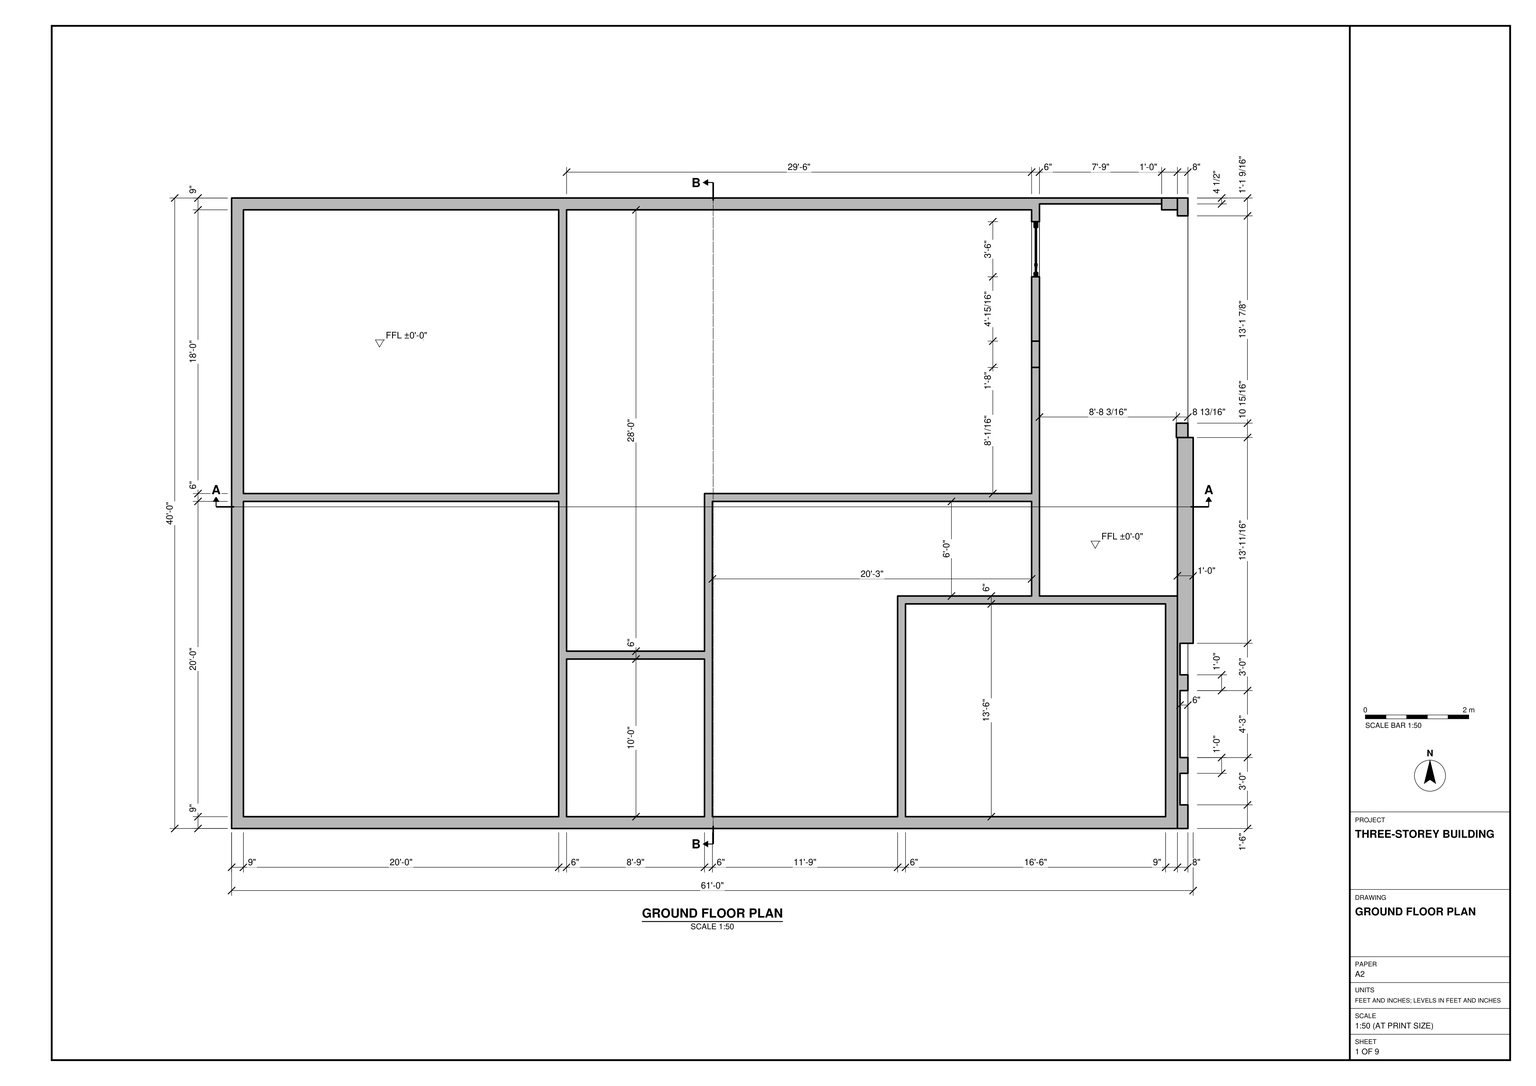
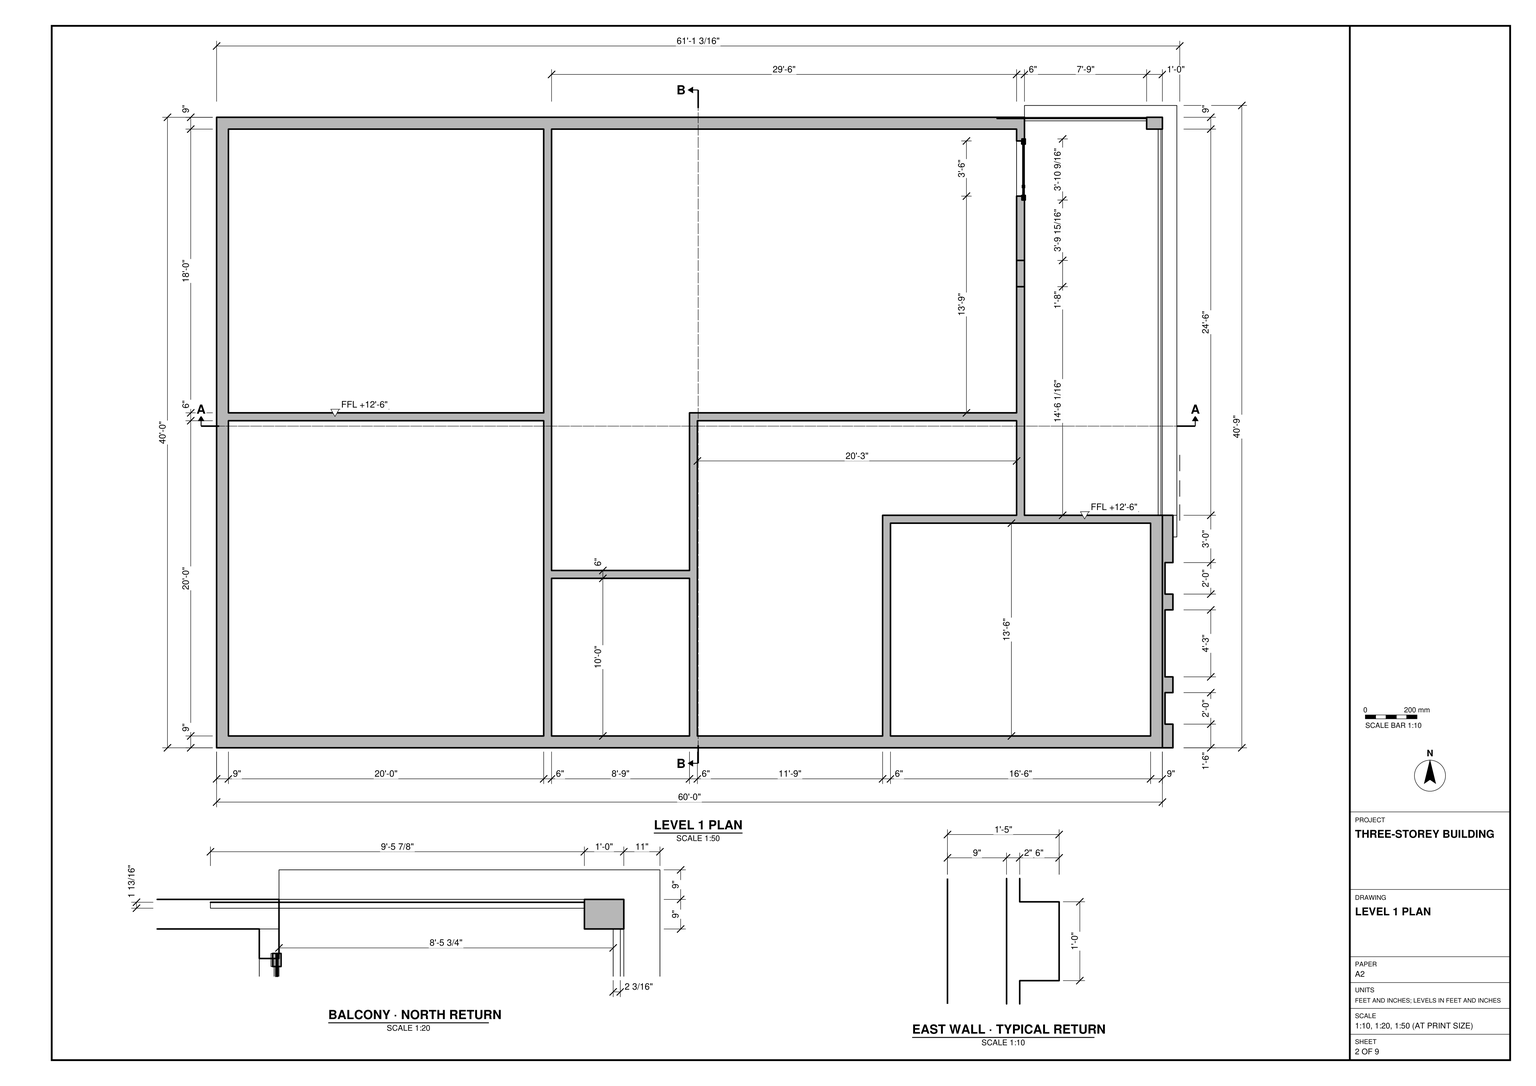
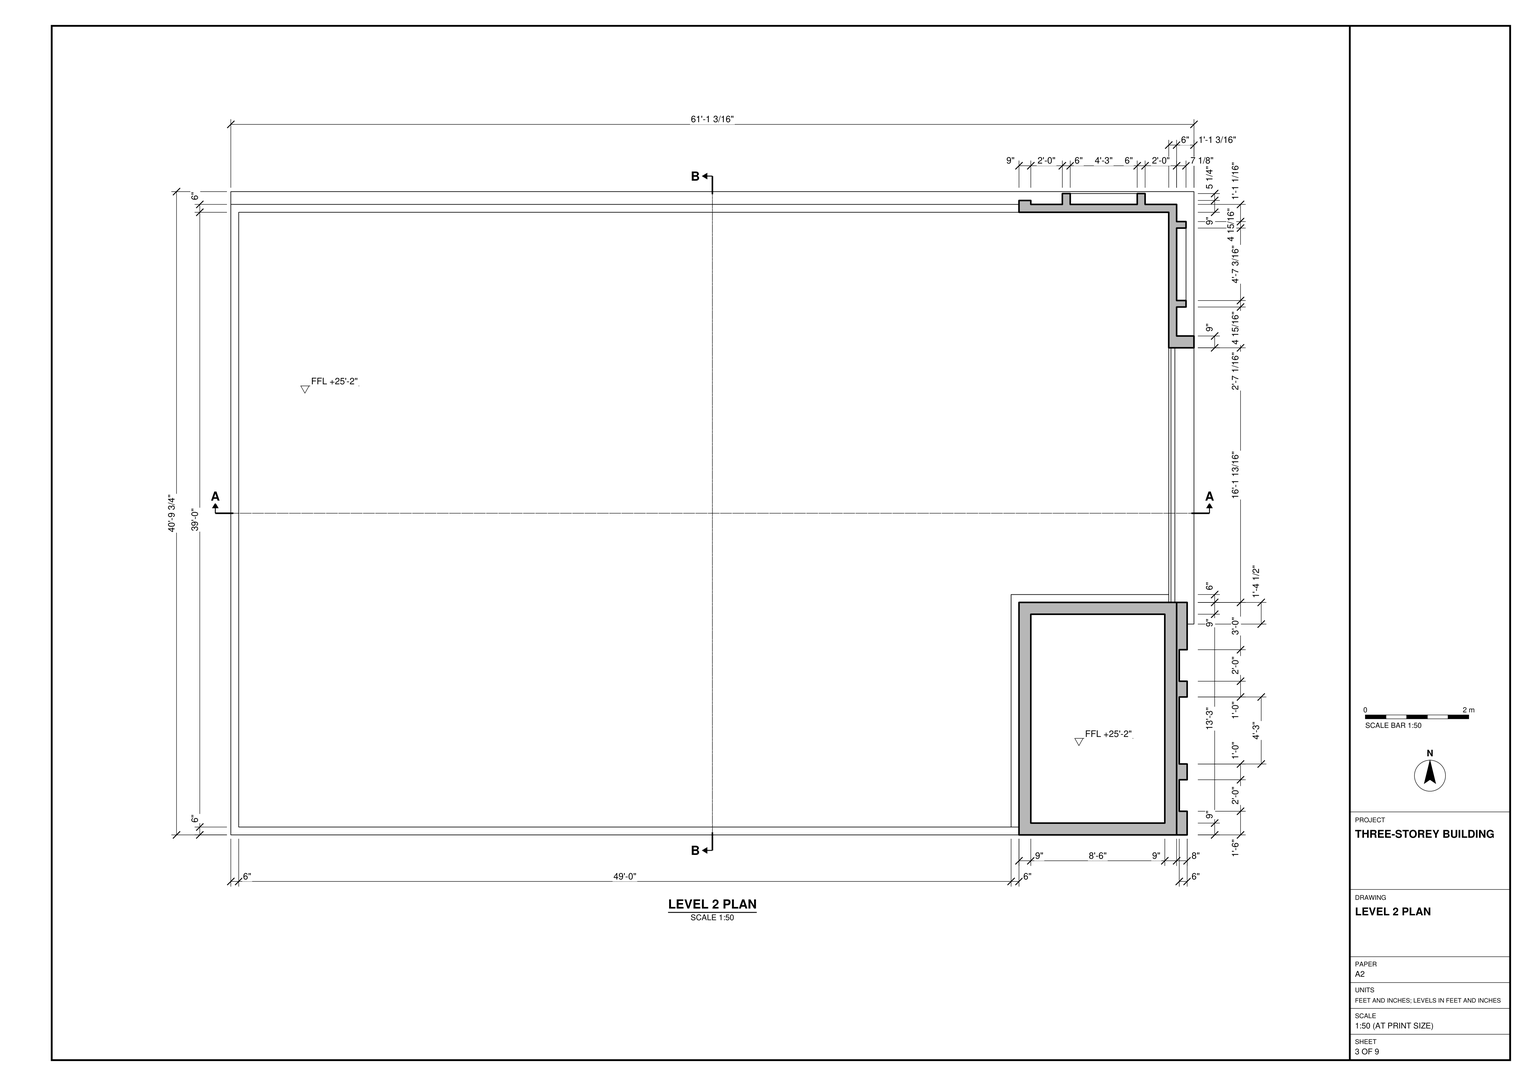
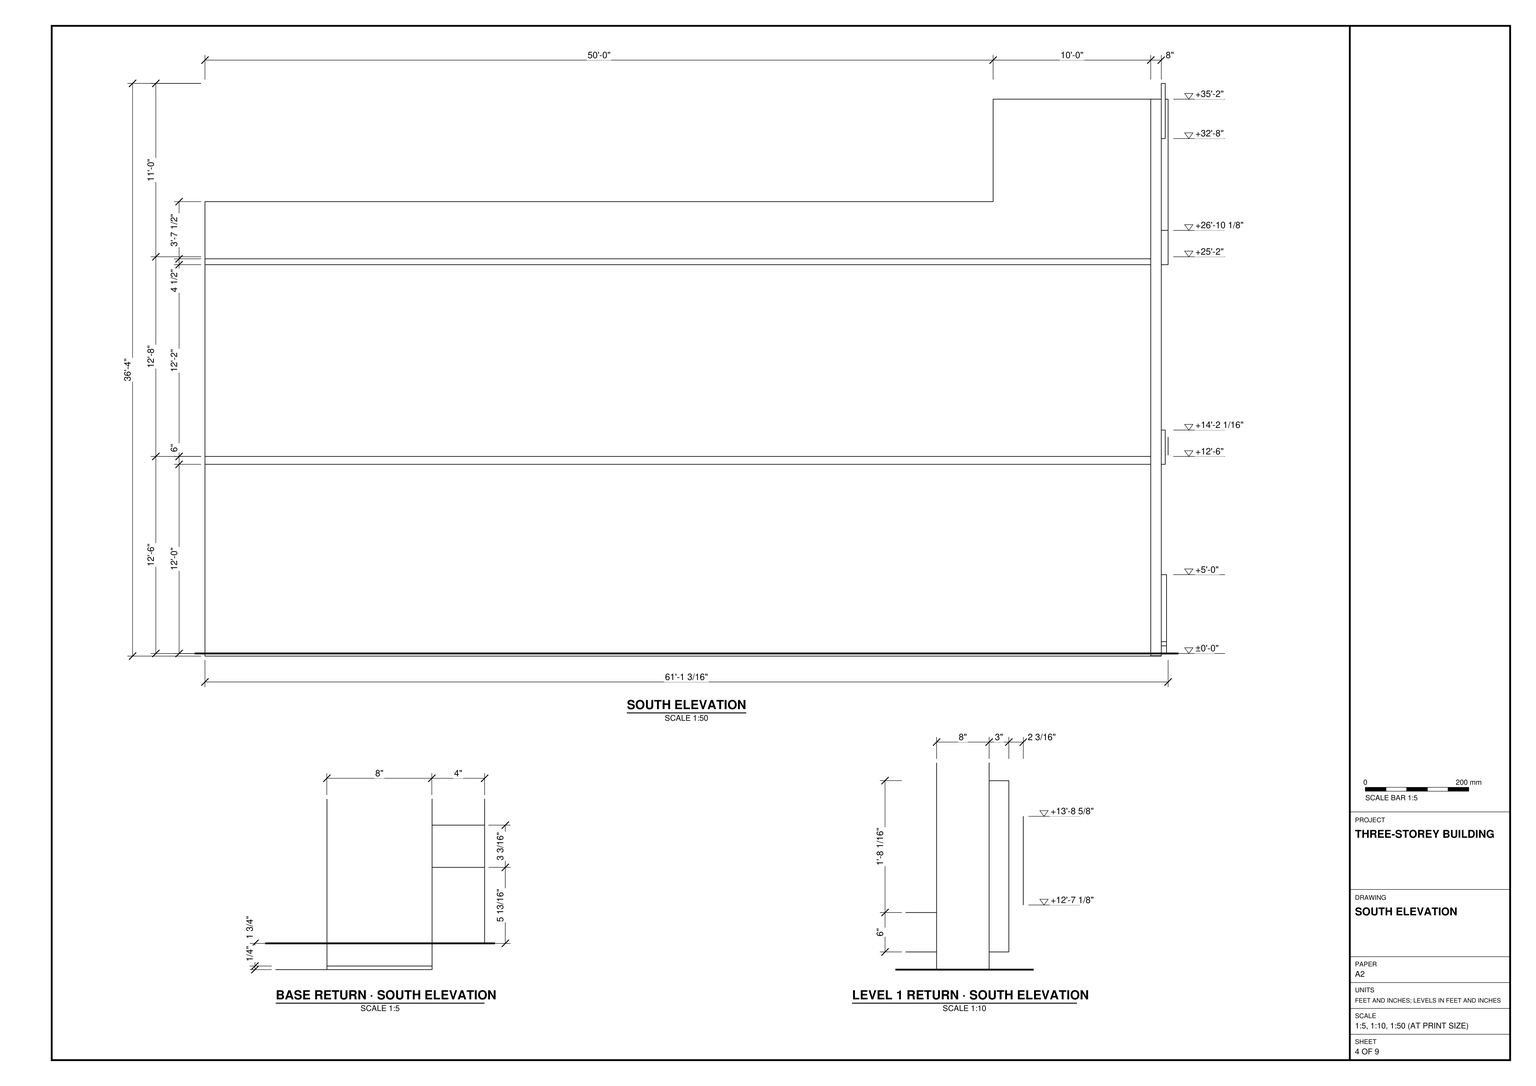
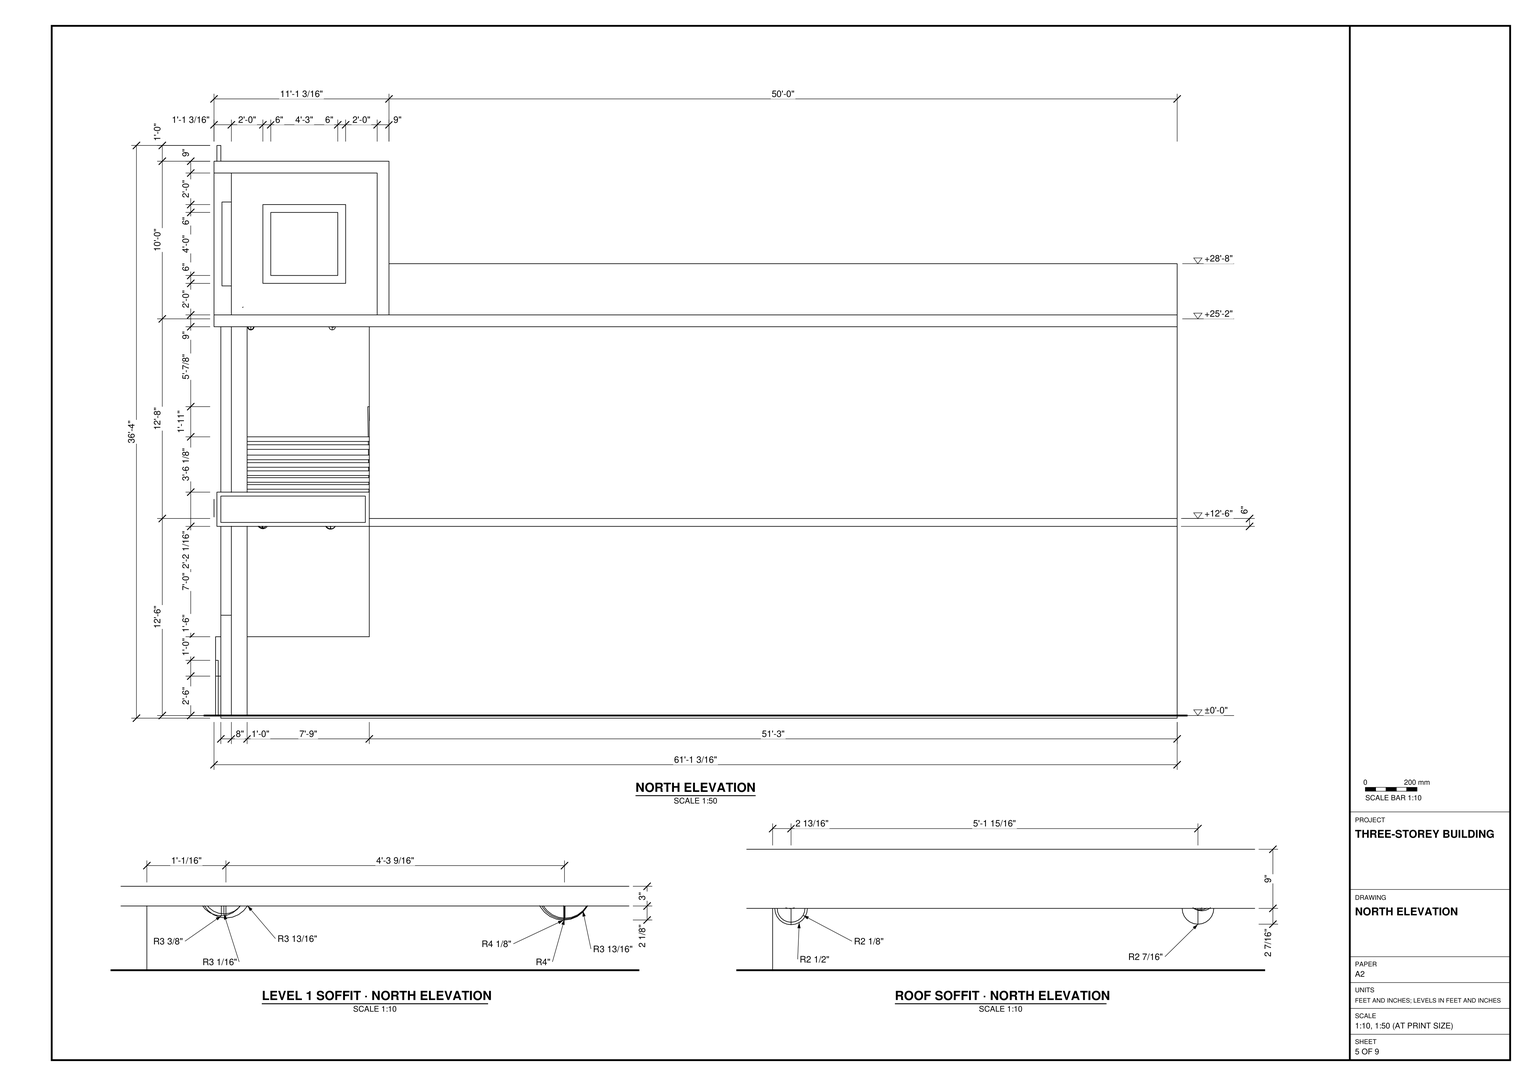
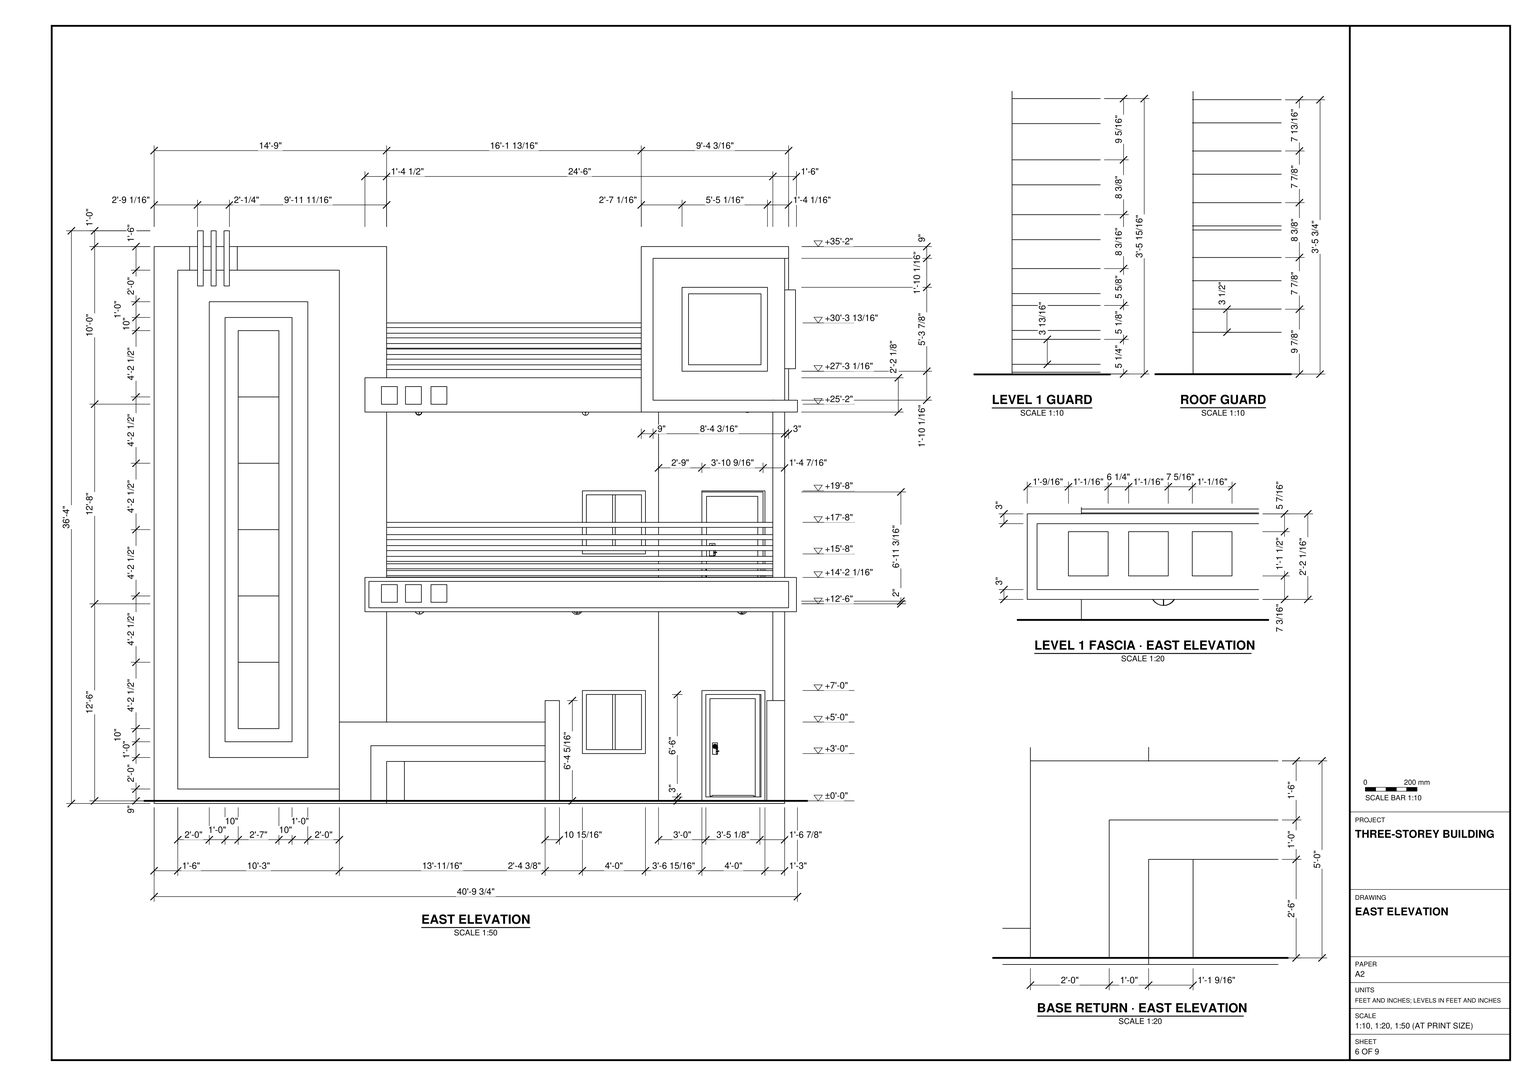
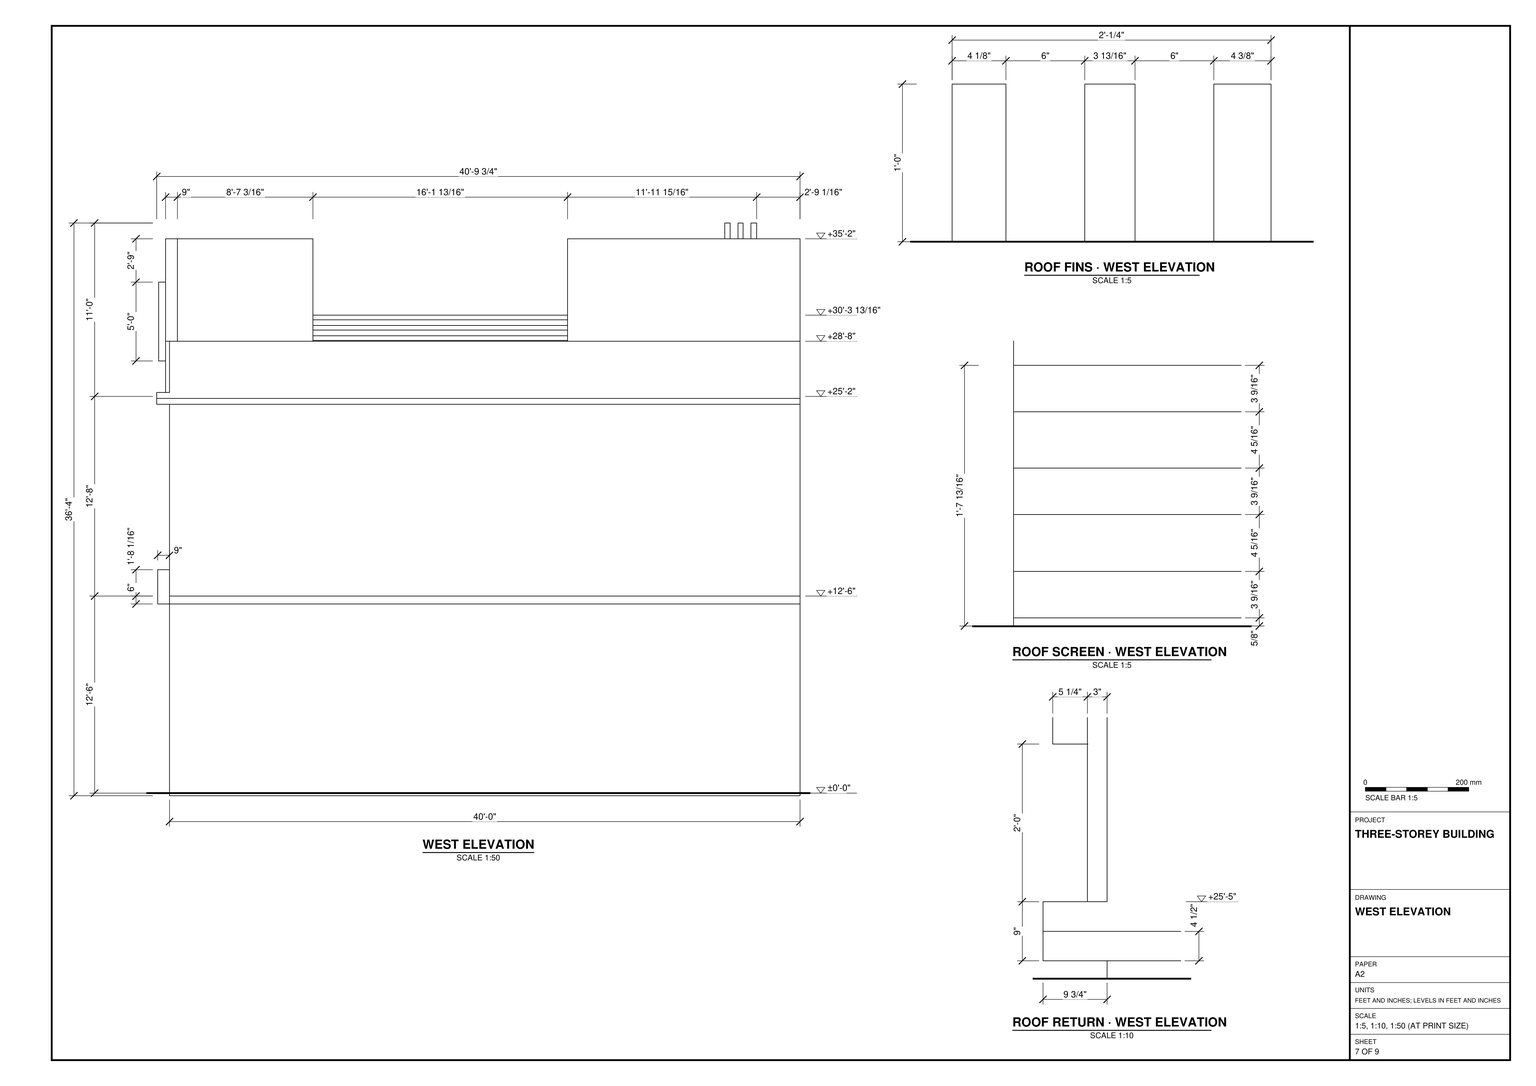
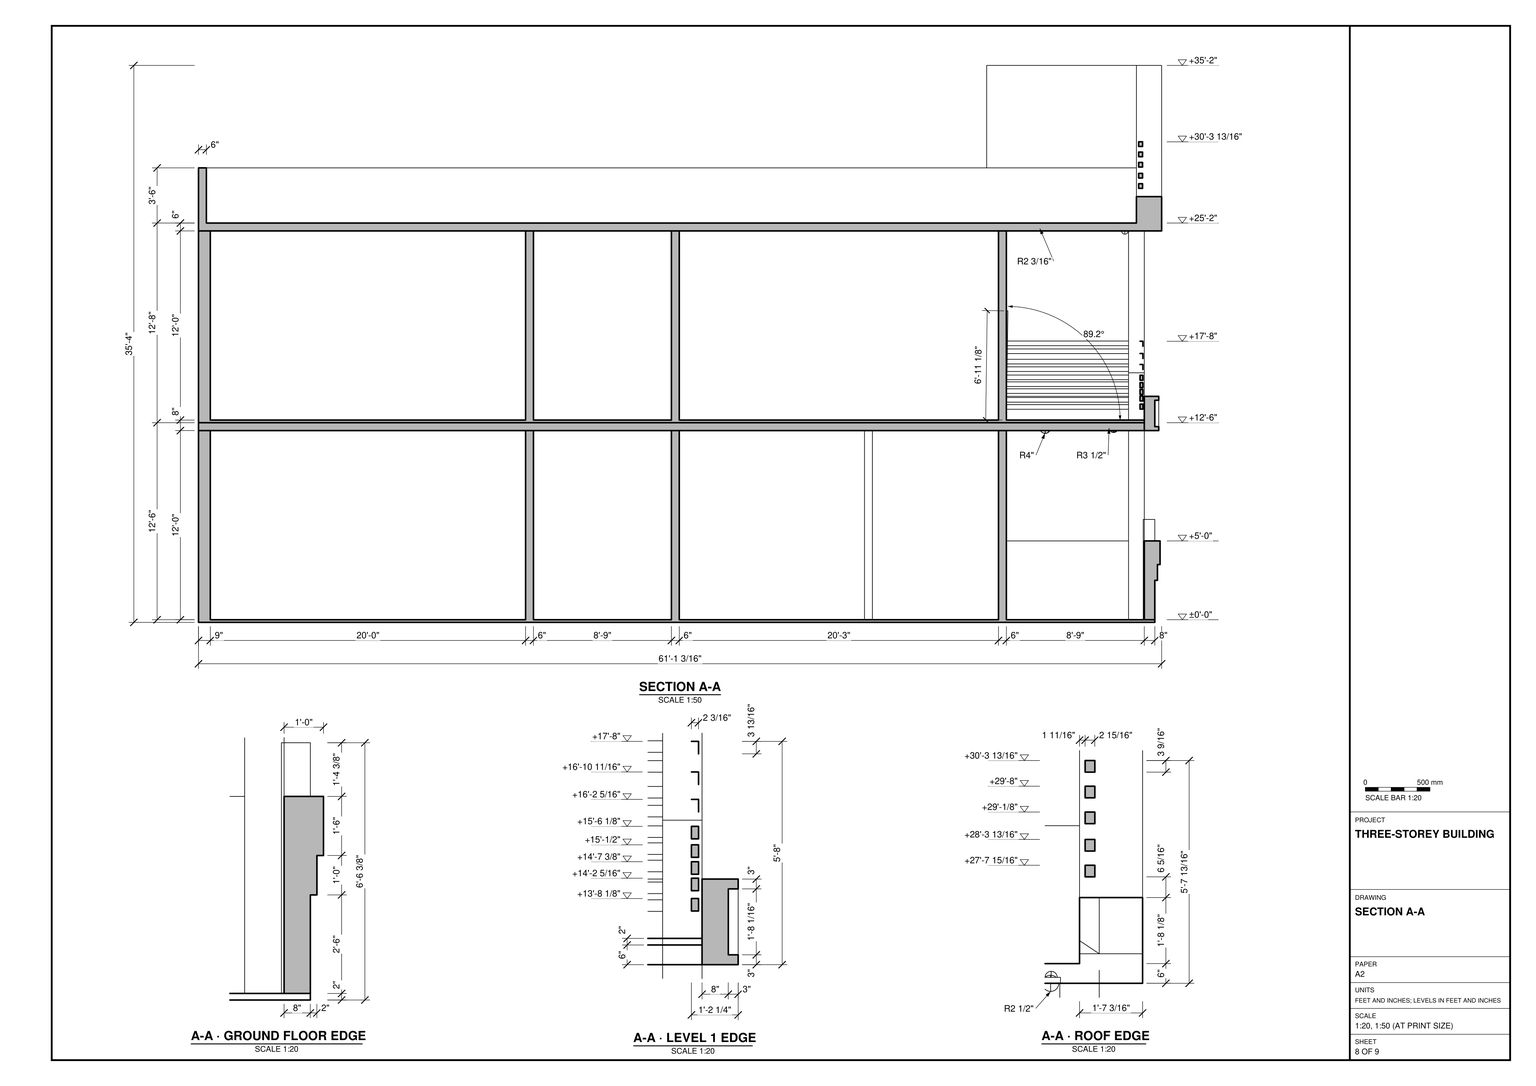
Use task_files/diagram_01.pdf to build the three-storey building in SketchUp. Work in feet and inches. Orient the plans with north at the top. The finished model measures 61'-1 3/16" east to west, 40'-9 3/4" north to south and 36'-4" in height. Set the finished floor levels to ±0'-0", +12'-6" and +25'-2".

Lay out the ground floor and Level 1 from their respective plans. Match the two large western rooms, the narrow south-central room and the stepped partitions around the southeast room. Use the wall thicknesses marked on the plans, including the 9" perimeter walls and 6" partitions where indicated. Form the openings in the walls and fit the door and window units where shown. Model the floor slabs and the recessed east bay, distinguishing the ground-floor edge from the balcony above it. Use the balcony north-return detail and the east-wall return detail to shape those edges.

Keep most of Level 2 open as a roof terrace. Model its perimeter, the small southeast enclosure and its roof, and the stepped wall at the northeast corner. Follow the sheets for any stairs, built-in joinery and main furniture shown. Any decor or loose items shown may be suitable library components. Keep walls, slabs, roof elements and individual furniture or joinery pieces in separate groups or components, and use components for repeated parts. Save one SketchUp model as output_files/three_storey_building_with_balcony_and_roof_terrace.skp.

# SketchUp Ruby script. Lengths in inches.
U = 1.inch
M = Sketchup.active_model
def pt(a) = Geom::Point3d.new(a.map { |v| v * U })
def face(e, loops, mat)
  f = e.add_face(loops[0].map { |a| pt(a) })
  loops[1..].each { |l| e.add_face(l.map { |a| pt(a) }).erase! }
  f.material = f.back_material = mat if mat
  f
end
# faces: each face lists its corners as indices into pts; further lists are holes
def faces(e, pts, list, mat = nil) = list.each { |f| face(e, (f[0].is_a?(Array) ? f : [f]).map { |l| l.map { |i| pts[i] } }, mat) }
# xy, xz, yz: faces in a plane at the given z, y or x. An outline is a flat list of corners, or four numbers for a rectangle; further outlines are holes
def ring(l) = l.size == 4 ? [[l[0], l[1]], [l[2], l[1]], [l[2], l[3]], [l[0], l[3]]] : l.each_slice(2).to_a
def flat(e, list, mat, &to3) = list.each { |f| face(e, (f[0].is_a?(Array) ? f : [f]).map { |l| ring(l).map { |u, v| to3.(u, v) } }, mat) }
def xy(e, z, list, mat = nil) = flat(e, list, mat) { |x, y| [x, y, z] }
def xz(e, y, list, mat = nil) = flat(e, list, mat) { |x, z| [x, y, z] }
def yz(e, x, list, mat = nil) = flat(e, list, mat) { |y, z| [x, y, z] }
def lines(e, pts, list) = list.each { |a, b| e.add_line(pt(pts[a]), pt(pts[b])) }
# prism: a flat outline (further loops are holes) pulled along v
def prism(e, loops, v, mat = nil)
  f = face(e, loops, mat); d = Geom::Vector3d.new(v.map { |x| x * U })
  f.pushpull(f.normal.samedirection?(d) ? d.length : -d.length)
end
def box(e, o, s, mat = nil) = prism(e, [[o, [o[0] + s[0], o[1], o[2]], [o[0] + s[0], o[1] + s[1], o[2]], [o[0], o[1] + s[1], o[2]]]], [0, 0, s[2]], mat)
def at(x, y, z, deg = 0) = Geom::Transformation.translation(pt([x, y, z])) * Geom::Transformation.rotation(ORIGIN, Z_AXIS, deg.degrees)
def axes(o, x, y, z) = Geom::Transformation.new([*x, 0, *y, 0, *z, 0, *pt(o).to_a, 1])
def part(name) = M.definitions.add(name)
# library, detail: a bought-in or finely detailed component or shape, given as its bounding box
def library(name, o, s) = part(name).tap { |d| box(d.entities, o, s) }
def detail(e, o, s) = box(e.add_group.entities, o, s)
def put(e, d, t, mat = nil) = e.add_instance(d, t).tap { |i| i.material = mat if mat }
def group(e, t, mat = nil) = e.add_group.tap { |g| g.transformation = t; g.material = mat if mat }.entities
root = M.entities
M.materials.add("D01_Frost_White").color = [255, 242, 206]
M.materials.add("D03_Lemon_Mist").color = [255, 216, 101]
M.materials.add("Glass_Mirror_01").color = [185, 185, 185]
M.materials.add("Metal_10_1K").color = [196, 175, 123]
M.materials.add("Plywood_01_1K").color = [125, 96, 64]
M.materials.add("Roofing_01_1K").color = [84, 79, 73]
M.materials.add("ThomThom - Beard1").color = [168, 140, 112]
M.materials.add("ThomThom - Complexion1").color = [237, 210, 184]
M.materials.add("Wood_Veneer_15_1K").color = [103, 69, 45]
c1 = library("porta+4",[0.2,-5.42,1.33],[46.55,4.72,83.21])
c2 = library("Group\#4",[0,0,-2.15],[720,480,8.29])
c3 = library("Group\#2",[0,0,-296],[733.2,489.76,422])
xy(root,2,[[720,0,720,297.66,728,297.66,728,190.54,730,190.54,730,165,732,165,732,141,728,141,728,0],[9,9,249,249],[255,9,360,129],[366,9,507,9,507,177,609,177,609,249,366,249],[513,9,711,171],
  [9,255,249,471],[719.19,297.66,728,308.57],[720,466.42,728,480]])
xy(root,11,[[722,18,728,141]])
xy(root,32,[[728,190.54,730,297.66]],"ThomThom - Beard1")
xy(root,35,[[722,42,728,117]])
xy(root,41,[[609,351.03,615,371.03]])
xy(root,44,[[730,165,732,297.66]],"Roofing_01_1K")
xy(root,47,[[722,54,728,105]])
xy(root,62,[[728,141,732,141,732,297.66,720,297.66,720,177,728,177]])
xy(root,78.34,[[719.19,297.66,728,308.57],[720,466.42,728,480]],"Plywood_01_1K")
xy(root,83,[[609,351.03,615,371.03]])
xy(root,146,[[720,177,720,480.02,615,480.02,615,489,731,489,731,177]])
xy(root,146,[[728,160.5,731,177]],"ThomThom - Complexion1")
xy(root,149,[[728,163.5,731,177],[728,177,731,483],[618,486,728,489]],"ThomThom - Complexion1")
xy(root,162.23,[[615,477.3125,708,479.11]])
xy(root,165.75,[[615,477.3125,708,479.11]],"Wood_Veneer_15_1K")
xy(root,167.64,[[615,477.3125,708,479.11]])
xy(root,169.07,[[728,163.5,731,177],[728,177,731,483],[618,486,728,489]],"ThomThom - Complexion1")
xy(root,171.16,[[615,477.3125,708,479.11]],"Wood_Veneer_15_1K")
xy(root,172.07,[[720,177,731,177,731,489,615,489,615,480.02,720,480.02]])
xy(root,172.07,[[728,160.5,731,177]],"ThomThom - Complexion1")
xy(root,174.29,[[615,477.3125,708,479.11]])
xy(root,177.81,[[615,477.3125,708,479.11]],"Wood_Veneer_15_1K")
xy(root,179.57,[[615,477.3125,708,479.11]])
xy(root,183.09,[[615,477.3125,708,479.11]],"Wood_Veneer_15_1K")
xy(root,184.75,[[594.11,477.3125,708,479.11]])
xy(root,188.27,[[594.11,477.3125,708,479.11]],"Wood_Veneer_15_1K")
xy(root,193,[[609,351.03,615,371.03]])
xy(root,235,[[609,351.03,615,371.03]])
xy(root,370,[[722,54,728,105]])
xy(root,382,[[722,42,728,117]])
xy(root,394,[[728,33.04,731,37.39],[728,43.39,731,47.22],[728,53.22,731,57.32]])
xy(root,406,[[722,18,728,141]])
xy(root,424,[[720,0,728,177]])
xy(root,436,[[728,33.04,731,37.39],[728,43.39,731,47.22],[728,53.22,731,57.32]],"Plywood_01_1K")
xz(root,0,[[720,2,728,424]])
xz(root,18,[[722,11,728,406]])
xz(root,33.04,[[728,394,731,436]],"Plywood_01_1K")
xz(root,37.39,[[728,394,731,436]],"Plywood_01_1K")
xz(root,42,[[722,35,728,382]])
xz(root,43.39,[[728,394,731,436]],"Plywood_01_1K")
xz(root,47.22,[[728,394,731,436]],"Plywood_01_1K")
xz(root,53.22,[[728,394,731,436]],"Plywood_01_1K")
xz(root,54,[[722,47,728,370]])
xz(root,57.32,[[728,394,731,436]],"Plywood_01_1K")
xz(root,105,[[722,47,728,146],[722,146,728,370]])
xz(root,117,[[722,35,728,146],[722,146,728,382]])
xz(root,141,[[722,11,732,11,732,62,728,62,728,146,722,146],[722,146,728,406]])
xz(root,141,[[728,2,732,7.79],[728,7.79,732,11]],"Roofing_01_1K")
xz(root,160.5,[[728,146,731,172.07]],"ThomThom - Complexion1")
xz(root,163.5,[[728,149,731,169.07]],"ThomThom - Complexion1")
xz(root,165,[[730,2,732,32],[730,32,732,44]],"Roofing_01_1K")
xz(root,177,[[720,62,728,146],[720,172.07,728,424]])
xz(root,190.54,[[728,2,730,32]],"Wood_Veneer_15_1K")
xz(root,297.66,[[719.19,2,720,78.34],[720,2,728,62],[728,32,728,62,732,62,732,44,730,44,730,32]])
xz(root,297.66,[[720,62,728,78.34]],"Plywood_01_1K")
xz(root,308.57,[[719.19,2,728,78.34]],"Plywood_01_1K")
xz(root,351.03,[[609,41,615,83],[609,193,615,235]])
xz(root,371.03,[[609,41,615,83],[609,193,615,235]])
xz(root,466.42,[[720,2,728,78.34]],"Plywood_01_1K")
xz(root,477.3125,[[615,162.23,708,165.75],[615,167.64,708,171.16],[615,174.29,708,177.81],[615,179.57,708,183.09],[594.11,184.75,708,188.27]])
xz(root,479.11,[[615,162.23,708,165.75],[615,167.64,708,171.16],[615,174.29,708,177.81],[615,179.57,708,183.09],[594.11,184.75,708,188.27],
  [594.11,191,708,194.52],[594.11,196.75,708,200.27],[594.11,204.61,708,208.13],[594.11,210.66,708,214.18]],"Wood_Veneer_15_1K")
xz(root,480,[[720,2,728,78.34]],"Plywood_01_1K")
xz(root,480.02,[[615,146,720,172.07]])
xz(root,483,[[728,149,731,169.07]],"ThomThom - Complexion1")
xz(root,486,[[618,149,728,169.07]],"ThomThom - Complexion1")
xz(root,489,[[[615,146,731,172.07],[618,149,728,169.07]]],"ThomThom - Complexion1")
yz(root,594.11,[[477.3125,184.75,479.11,188.27]])
yz(root,609,[[351.03,41,371.03,83],[351.03,193,371.03,235]])
yz(root,615,[[480.02,146,489,172.07],[477.3125,162.23,479.11,165.75],[477.3125,167.64,479.11,171.16],[477.3125,174.29,479.11,177.81],[477.3125,179.57,479.11,183.09]])
yz(root,618,[[486,149,489,169.07]],"ThomThom - Complexion1")
yz(root,708,[[477.3125,162.23,479.11,165.75],[477.3125,167.64,479.11,171.16],[477.3125,174.29,479.11,177.81],[477.3125,179.57,479.11,183.09],[477.3125,184.75,479.11,188.27]])
yz(root,719.19,[[297.66,2,308.57,78.34]])
yz(root,720,[[177,2,297.66,62],[466.42,2,480,78.34],[177,146,480.02,172.07]])
yz(root,722,[[64,57,95,107.5],[64,107.5,95,158],[64,158,95,208.5],[64,208.5,95,259],[64,259,95,309.5],
  [64,309.5,95,360]],"Metal_10_1K")
yz(root,722,[[[18,11,141,406],[42,35,117,382]]],"Plywood_01_1K")
yz(root,722,[[[54,47,105,370],[64,57,95,360]]],"ThomThom - Complexion1")
yz(root,728,[[33.04,394,37.39,406],[43.39,394,47.22,406],[53.22,394,57.32,406],[33.04,406,37.39,424],[43.39,406,47.22,424],
  [53.22,406,57.32,424],[33.04,424,37.39,436],[43.39,424,47.22,436],[53.22,424,57.32,436]])
yz(root,728,[[297.66,2,308.57,78.34],[466.42,2,480,78.34]],"Plywood_01_1K")
yz(root,728,[[0,2,141,2,141,11,18,11,18,406,27.04,406,27.04,424,0,424],[[42,35,117,382],[54,47,105,370]],[141,62,177,62,177,146,160.5,146,160.5,172.07,177,172.07,177,424,63.32,424,63.32,406,141,406],[27.04,406,33.04,424],[37.39,406,43.39,424],
  [47.22,406,53.22,424],[57.32,406,63.32,424]],"Roofing_01_1K")
yz(root,728,[[163.5,149,483,169.07],[486,149,489,169.07]],"ThomThom - Complexion1")
yz(root,728,[[190.54,2,297.66,32]],"Wood_Veneer_15_1K")
yz(root,730,[[165,2,177,2,177,32,297.66,32,297.66,44,165,44]],"ThomThom - Beard1")
yz(root,730,[[177,2,190.54,32]],"Wood_Veneer_15_1K")
yz(root,731,[[33.04,394,37.39,436],[43.39,394,47.22,436],[53.22,394,57.32,436]],"ThomThom - Beard1")
yz(root,731,[[[160.5,146,489,172.07],[163.5,149,483,169.07]]],"ThomThom - Complexion1")
yz(root,732,[[141,2,165,2,165,44,297.66,44,297.66,62,141,62]],"Roofing_01_1K")
# 35 loose lines left out
put(root,c1,axes([615.67,419.82,3.71],[0,0.88392,0],[0.96185,0,0],[0,0,0.93792]))
put(root,c1,at(610.72,416.8,152.66,90))
g1 = group(root,at(0,0,0),"ThomThom - Complexion1")
xy(g1,0,[[0,0,0,480,728,480,728,177,720,177,720,0]])
xy(g1,2,[[255,135,360,135,360,255,609,255,609,471,255,471],[615,177,728,177,728,480,708,480,708,475.5,615,475.5],[609,255,615,471]])
xy(g1,5,[[609,420,615,462]])
xy(g1,62,[[615,475.5,708,480]])
xy(g1,83,[[609,420,615,462]])
xy(g1,146,[[[0,0,720,0,720,177,615,177,615,480,0,480],[366,9,366,249,609,249,609,255,360,255,360,135,255,135,255,471,609,471,609,177,507,177,507,9],[9,9,249,249],[9,255,249,471],[513,9,711,171],[255,9,360,129]]])
xz(g1,0,[[0,0,720,146]])
xz(g1,9,[[9,2,249,146],[255,2,360,146],[366,2,507,146],[513,2,609,146],[609,2,615,146],
  [615,2,711,146]])
xz(g1,129,[[255,2,360,146]])
xz(g1,135,[[255,2,360,146]])
xz(g1,171,[[513,2,609,146],[609,2,615,146],[615,2,711,146]])
xz(g1,177,[[720,0,728,0.27],[720,0.27,728,2],[507,2,609,146],[711,2,720,146]])
xz(g1,177,[[615,2,711,146]],"D03_Lemon_Mist")
xz(g1,249,[[9,2,249,146],[366,2,507,146],[507,2,513,146],[513,2,609,146]])
xz(g1,255,[[9,2,249,146],[360,2,609,146]])
xz(g1,420,[[609,5,615,83]])
xz(g1,462,[[609,5,615,83]])
xz(g1,471,[[9,2,249,146],[255,2,609,146]])
xz(g1,475.5,[[615,2,708,62]])
xz(g1,480,[[0,0,0,146,615,146,615,62,708,62,708,2,728,2,728,0]])
yz(g1,0,[[0,0,480,146]])
yz(g1,9,[[9,2,249,146],[255,2,471,146]])
yz(g1,249,[[9,2,249,146],[255,2,471,146]])
yz(g1,255,[[9,2,129,146],[135,2,471,146]])
yz(g1,360,[[9,2,129,146],[135,2,255,146]])
yz(g1,366,[[9,2,249,146]])
yz(g1,507,[[9,2,177,146]])
yz(g1,513,[[9,2,171,146]])
yz(g1,609,[[177,2,249,146],[[255,2,471,146],[420,5,462,83]]])
yz(g1,615,[[[417,2,465,86],[420,5,462,83]]])
yz(g1,615,[[[177,2,384,146],[326.03,38,374.03,86]]],"D01_Frost_White")
yz(g1,615,[[329.03,41,349.03,83],[351.03,41,371.03,83]],"Glass_Mirror_01")
yz(g1,615,[[384,2,417,2,417,86,465,86,465,2,475.5,2,475.5,62,480,62,480,146,384,146],[[326.03,38,374.03,86],[329.03,41,349.03,83],[351.03,41,371.03,83]]],"Wood_Veneer_15_1K")
yz(g1,708,[[475.5,2,480,62]])
yz(g1,711,[[9,2,171,146]])
yz(g1,720,[[0,0,177,146]])
yz(g1,728,[[177,0,480,2]])
# 1 loose lines left out
put(root,c2,at(0,0,146),"ThomThom - Complexion1")
g2 = group(root,at(0,0,152),"ThomThom - Complexion1")
xy(g2,0,[[0,0,720,480]])
xy(g2,2,[[9,9,249,249],[255,9,360,129],[366,9,507,9,507,177,609,177,609,249,366,249],[513,9,711,171],[255,135,360,135,360,255,609,255,609,471,255,471],
  [615,177,720,480],[9,255,249,471],[609,255,615,471]])
xy(g2,5,[[609,420,615,462]])
xy(g2,83,[[609,420,615,462]])
xz(g2,0,[[0,0,720,146]])
xz(g2,9,[[9,2,249,146],[255,2,360,146],[366,2,507,146],[513,2,711,146]])
xz(g2,129,[[255,2,360,146]])
xz(g2,135,[[255,2,360,146]])
xz(g2,171,[[513,2,711,146]])
xz(g2,177,[[507,2,609,146]])
xz(g2,177,[[615,2,720,146]],"D03_Lemon_Mist")
xz(g2,249,[[9,2,249,146],[366,2,609,146]])
xz(g2,255,[[9,2,249,146],[360,2,609,146]])
xz(g2,420,[[609,5,615,83]])
xz(g2,462,[[609,5,615,83]])
xz(g2,471,[[9,2,249,146],[255,2,609,146]])
xz(g2,480,[[0,0,0,146,615,146,615,2,720,2,720,0]])
yz(g2,0,[[0,0,480,146]])
yz(g2,9,[[9,2,249,146],[255,2,471,146]])
yz(g2,249,[[9,2,249,146],[255,2,471,146]])
yz(g2,255,[[9,2,129,146],[135,2,471,146]])
yz(g2,360,[[9,2,129,146],[135,2,255,146]])
yz(g2,366,[[9,2,249,146]])
yz(g2,507,[[9,2,177,146]])
yz(g2,513,[[9,2,171,146]])
yz(g2,609,[[177,2,249,146],[[255,2,471,146],[420,5,462,83]]])
yz(g2,615,[[[417,2,465,86],[420,5,462,83]]])
yz(g2,615,[[[177,2,384,146],[326.03,38,374.03,86]]],"D01_Frost_White")
yz(g2,615,[[329.03,41,349.03,83],[351.03,41,371.03,83]],"Glass_Mirror_01")
yz(g2,615,[[384,2,417,2,417,86,465,86,465,2,480,2,480,146,384,146],[[326.03,38,374.03,86],[329.03,41,349.03,83],[351.03,41,371.03,83]]],"Wood_Veneer_15_1K")
yz(g2,711,[[9,2,171,146]])
yz(g2,720,[[0,0,480,0,480,2,177,2,177,146,0,146]])
# 2 loose lines left out
put(root,c3,at(0,0,298),"ThomThom - Complexion1")
